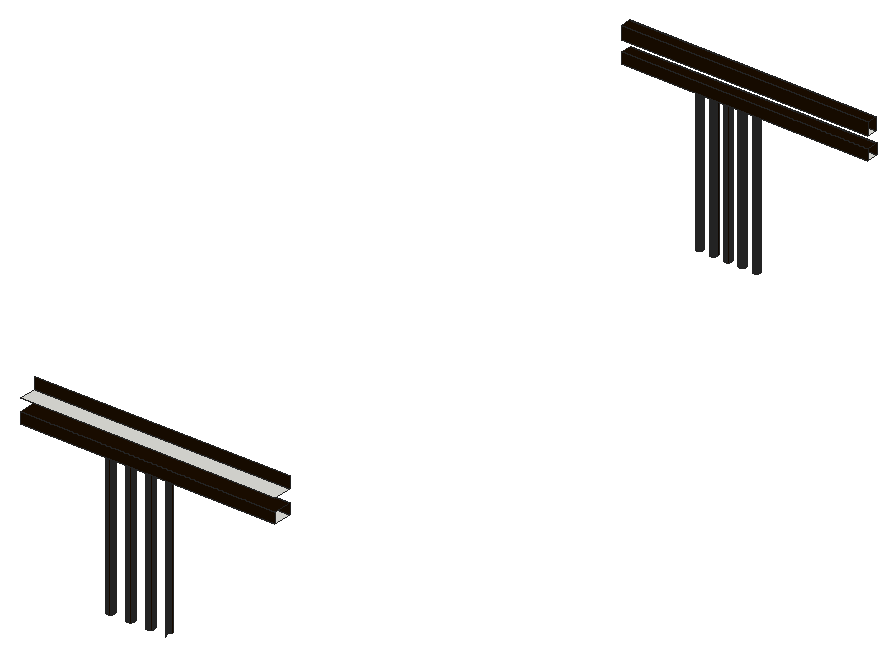
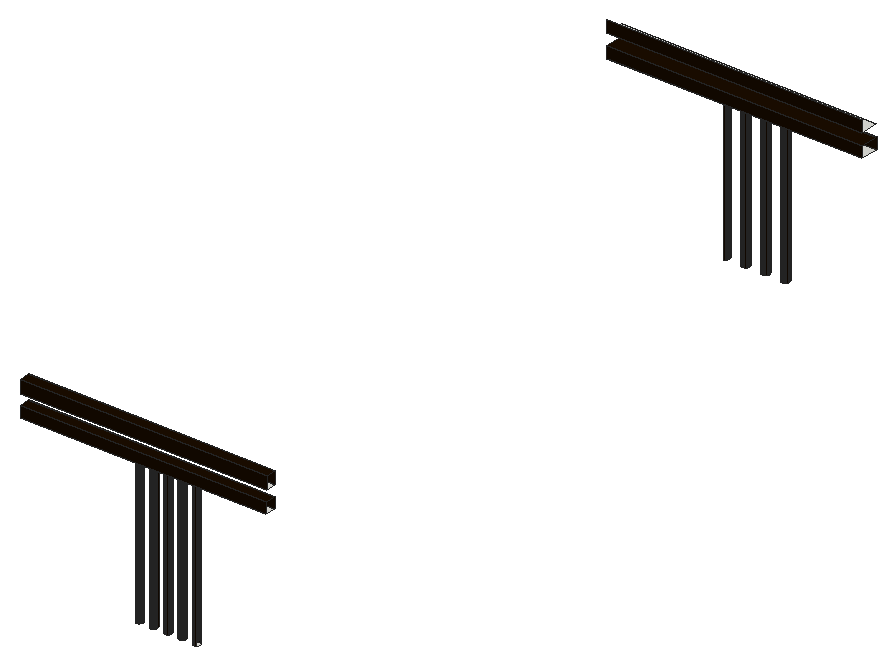
# SketchUp Ruby script. Lengths in inches.
U = 1.inch
M = Sketchup.active_model
def pt(a) = Geom::Point3d.new(a.map { |v| v * U })
def face(e, loops, mat)
  f = e.add_face(loops[0].map { |a| pt(a) })
  loops[1..].each { |l| e.add_face(l.map { |a| pt(a) }).erase! }
  f.material = f.back_material = mat if mat
  f
end
# faces: each face lists its corners as indices into pts; further lists are holes
def faces(e, pts, list, mat = nil) = list.each { |f| face(e, (f[0].is_a?(Array) ? f : [f]).map { |l| l.map { |i| pts[i] } }, mat) }
# xy, xz, yz: faces in a plane at the given z, y or x. An outline is a flat list of corners, or four numbers for a rectangle; further outlines are holes
def ring(l) = l.size == 4 ? [[l[0], l[1]], [l[2], l[1]], [l[2], l[3]], [l[0], l[3]]] : l.each_slice(2).to_a
def flat(e, list, mat, &to3) = list.each { |f| face(e, (f[0].is_a?(Array) ? f : [f]).map { |l| ring(l).map { |u, v| to3.(u, v) } }, mat) }
def xy(e, z, list, mat = nil) = flat(e, list, mat) { |x, y| [x, y, z] }
def xz(e, y, list, mat = nil) = flat(e, list, mat) { |x, z| [x, y, z] }
def yz(e, x, list, mat = nil) = flat(e, list, mat) { |y, z| [x, y, z] }
def lines(e, pts, list) = list.each { |a, b| e.add_line(pt(pts[a]), pt(pts[b])) }
# prism: a flat outline (further loops are holes) pulled along v
def prism(e, loops, v, mat = nil)
  f = face(e, loops, mat); d = Geom::Vector3d.new(v.map { |x| x * U })
  f.pushpull(f.normal.samedirection?(d) ? d.length : -d.length)
end
def box(e, o, s, mat = nil) = prism(e, [[o, [o[0] + s[0], o[1], o[2]], [o[0] + s[0], o[1] + s[1], o[2]], [o[0], o[1] + s[1], o[2]]]], [0, 0, s[2]], mat)
def at(x, y, z, deg = 0) = Geom::Transformation.translation(pt([x, y, z])) * Geom::Transformation.rotation(ORIGIN, Z_AXIS, deg.degrees)
def axes(o, x, y, z) = Geom::Transformation.new([*x, 0, *y, 0, *z, 0, *pt(o).to_a, 1])
def part(name) = M.definitions.add(name)
# library, detail: a bought-in or finely detailed component or shape, given as its bounding box
def library(name, o, s) = part(name).tap { |d| box(d.entities, o, s) }
def detail(e, o, s) = box(e.add_group.entities, o, s)
def put(e, d, t, mat = nil) = e.add_instance(d, t).tap { |i| i.material = mat if mat }
def group(e, t, mat = nil) = e.add_group.tap { |g| g.transformation = t; g.material = mat if mat }.entities
root = M.entities
M.materials.add("[Metal Seamed]1").color = [28, 14, 0]
xy(root,618.25,[[304.26,68.79,303.92,68.83,303.61,68.97,303.33,69.17,303.125,69.45,302.99,69.76,302.95,70.1,302.99,70.44,303.125,70.76,303.33,71.03,303.61,71.24,303.92,71.37,304.26,71.41,304.6,71.37,304.92,71.24,305.19,71.03,305.4,70.76,305.53,70.44,305.57,70.1,305.53,69.76,305.4,69.45,305.19,69.17,304.92,68.97,304.6,68.83],[310.95,68.79,310.61,68.83,310.29,68.97,310.02,69.17,309.8125,69.45,309.68,69.76,309.64,70.1,309.68,70.44,309.8125,70.76,310.02,71.03,310.29,71.24,310.61,71.37,310.95,71.41,311.29,71.37,311.61,71.24,311.88,71.03,312.09,70.76,312.22,70.44,312.26,70.1,312.22,69.76,312.09,69.45,311.88,69.17,311.61,68.97,311.29,68.83],[303.33,318.74,303.05,318.8125,302.79,318.95,302.57,319.15,302.42,319.4,302.34,319.6875,302.33,319.98,302.4,320.27,302.54,320.52,302.74,320.74,302.99,320.89,303.27,320.97,303.57,320.98,303.85,320.91,304.11,320.77,304.32,320.57,304.48,320.32,304.56,320.04,304.57,319.74,304.5,319.46,304.36,319.2,304.16,318.99,303.91,318.83,303.625,318.75],[308.14,318.74,307.86,318.8125,307.6,318.95,307.39,319.15,307.23,319.4,307.15,319.6875,307.14,319.98,307.21,320.27,307.35,320.52,307.55,320.74,307.8,320.89,308.09,320.97,308.38,320.98,308.66,320.91,308.92,320.77,309.14,320.57,309.29,320.32,309.37,320.04,309.38,319.74,309.3125,319.46,309.17,319.2,308.97,318.99,308.72,318.83,308.4375,318.75],[312.96,318.74,312.67,318.8125,312.41,318.95,312.2,319.15,312.05,319.4,311.96,319.6875,311.96,319.98,312.02,320.27,312.16,320.52,312.37,320.74,312.62,320.89,312.9,320.97,313.19,320.98,313.48,320.91,313.74,320.77,313.95,320.57,314.1,320.32,314.19,320.04,314.19,319.74,314.125,319.46,313.98,319.2,313.78,318.99,313.53,318.83,313.25,318.75],
  [317.77,318.74,317.48,318.8125,317.23,318.95,317.01,319.15,316.86,319.4,316.78,319.6875,316.77,319.98,316.84,320.27,316.98,320.52,317.18,320.74,317.43,320.89,317.71,320.97,318,320.98,318.29,320.91,318.55,320.77,318.76,320.57,318.91,320.32,319,320.04,319.01,319.74,318.9375,319.46,318.8,319.2,318.59,318.99,318.34,318.83,318.0625,318.75],[322.58,318.74,322.3,318.8125,322.04,318.95,321.82,319.15,321.67,319.4,321.59,319.6875,321.58,319.98,321.65,320.27,321.79,320.52,321.99,320.74,322.24,320.89,322.52,320.97,322.82,320.98,323.1,320.91,323.36,320.77,323.57,320.57,323.73,320.32,323.81,320.04,323.82,319.74,323.75,319.46,323.61,319.2,323.41,318.99,323.16,318.83,322.875,318.75]])
xy(root,666.66,[[[275.92,67.16,361.98,73.28],[284.2,68.79,284.54,68.83,284.86,68.97,285.13,69.17,285.34,69.45,285.47,69.76,285.51,70.1,285.47,70.44,285.34,70.76,285.13,71.03,284.86,71.24,284.54,71.37,284.2,71.41,283.86,71.37,283.54,71.24,283.27,71.03,283.0625,70.76,282.93,70.44,282.89,70.1,282.93,69.76,283.0625,69.45,283.27,69.17,283.54,68.97,283.86,68.83],[290.89,68.79,291.23,68.83,291.54,68.97,291.81,69.17,292.02,69.45,292.15,69.76,292.2,70.1,292.15,70.44,292.02,70.76,291.81,71.03,291.54,71.24,291.23,71.37,290.89,71.41,290.55,71.37,290.23,71.24,289.96,71.03,289.75,70.76,289.62,70.44,289.57,70.1,289.62,69.76,289.75,69.45,289.96,69.17,290.23,68.97,290.55,68.83],[297.57,68.79,297.91,68.83,298.23,68.97,298.5,69.17,298.71,69.45,298.84,69.76,298.89,70.1,298.84,70.44,298.71,70.76,298.5,71.03,298.23,71.24,297.91,71.37,297.57,71.41,297.23,71.37,296.92,71.24,296.65,71.03,296.4375,70.76,296.31,70.44,296.26,70.1,296.31,69.76,296.4375,69.45,296.65,69.17,296.92,68.97,297.23,68.83],[304.26,68.79,304.6,68.83,304.92,68.97,305.19,69.17,305.4,69.45,305.53,69.76,305.57,70.1,305.53,70.44,305.4,70.76,305.19,71.03,304.92,71.24,304.6,71.37,304.26,71.41,303.92,71.37,303.61,71.24,303.33,71.03,303.125,70.76,302.99,70.44,302.95,70.1,302.99,69.76,303.125,69.45,303.33,69.17,303.61,68.97,303.92,68.83],[310.95,68.79,311.29,68.83,311.61,68.97,311.88,69.17,312.09,69.45,312.22,69.76,312.26,70.1,312.22,70.44,312.09,70.76,311.88,71.03,311.61,71.24,311.29,71.37,310.95,71.41,310.61,71.37,310.29,71.24,310.02,71.03,309.8125,70.76,309.68,70.44,309.64,70.1,309.68,69.76,309.8125,69.45,310.02,69.17,310.29,68.97,310.61,68.83],[324.32,68.79,324.66,68.83,324.98,68.97,325.25,69.17,325.46,69.45,325.59,69.76,325.64,70.1,325.59,70.44,325.46,70.76,325.25,71.03,324.98,71.24,324.66,71.37,324.32,71.41,323.98,71.37,323.67,71.24,323.4,71.03,323.1875,70.76,323.06,70.44,323.01,70.1,323.06,69.76,323.1875,69.45,323.4,69.17,323.67,68.97,323.98,68.83],[331.01,68.79,331.35,68.83,331.67,68.97,331.94,69.17,332.15,69.45,332.28,69.76,332.32,70.1,332.28,70.44,332.15,70.76,331.94,71.03,331.67,71.24,331.35,71.37,331.01,71.41,330.67,71.37,330.36,71.24,330.08,71.03,329.875,70.76,329.74,70.44,329.7,70.1,329.74,69.76,329.875,69.45,330.08,69.17,330.36,68.97,330.67,68.83],[351.89,68.79,352.23,68.83,352.55,68.97,352.82,69.17,353.03,69.45,353.16,69.76,353.2,70.1,353.16,70.44,353.03,70.76,352.82,71.03,352.55,71.24,352.23,71.37,351.89,71.41,351.55,71.37,351.23,71.24,350.96,71.03,350.75,70.76,350.62,70.44,350.58,70.1,350.62,69.76,350.75,69.45,350.96,69.17,351.23,68.97,351.55,68.83],[317.64,68.79,317.98,68.83,318.29,68.97,318.56,69.17,318.77,69.45,318.9,69.76,318.95,70.1,318.9,70.44,318.77,70.76,318.56,71.03,318.29,71.24,317.98,71.37,317.64,71.41,317.3,71.37,316.98,71.24,316.71,71.03,316.5,70.76,316.37,70.44,316.32,70.1,316.37,69.76,316.5,69.45,316.71,69.17,316.98,68.97,317.3,68.83]],[[278.88,317.52,361.98,321.28],[351.46,318.74,351.75,318.75,352.03,318.83,352.28,318.99,352.48,319.2,352.625,319.46,352.69,319.74,352.69,320.04,352.6,320.32,352.45,320.57,352.24,320.77,351.98,320.91,351.69,320.98,351.4,320.97,351.12,320.89,350.87,320.74,350.66,320.52,350.52,320.27,350.46,319.98,350.46,319.6875,350.55,319.4,350.7,319.15,350.91,318.95,351.17,318.8125],[322.58,318.74,322.875,318.75,323.16,318.83,323.41,318.99,323.61,319.2,323.75,319.46,323.82,319.74,323.81,320.04,323.73,320.32,323.57,320.57,323.36,320.77,323.1,320.91,322.82,320.98,322.52,320.97,322.24,320.89,321.99,320.74,321.79,320.52,321.65,320.27,321.58,319.98,321.59,319.6875,321.67,319.4,321.82,319.15,322.04,318.95,322.3,318.8125],[317.77,318.74,318.0625,318.75,318.34,318.83,318.59,318.99,318.8,319.2,318.9375,319.46,319.01,319.74,319,320.04,318.91,320.32,318.76,320.57,318.55,320.77,318.29,320.91,318,320.98,317.71,320.97,317.43,320.89,317.18,320.74,316.98,320.52,316.84,320.27,316.77,319.98,316.78,319.6875,316.86,319.4,317.01,319.15,317.23,318.95,317.48,318.8125],[312.96,318.74,313.25,318.75,313.53,318.83,313.78,318.99,313.98,319.2,314.125,319.46,314.19,319.74,314.19,320.04,314.1,320.32,313.95,320.57,313.74,320.77,313.48,320.91,313.19,320.98,312.9,320.97,312.62,320.89,312.37,320.74,312.16,320.52,312.02,320.27,311.96,319.98,311.96,319.6875,312.05,319.4,312.2,319.15,312.41,318.95,312.67,318.8125],[308.14,318.74,308.4375,318.75,308.72,318.83,308.97,318.99,309.17,319.2,309.3125,319.46,309.38,319.74,309.37,320.04,309.29,320.32,309.14,320.57,308.92,320.77,308.66,320.91,308.38,320.98,308.09,320.97,307.8,320.89,307.55,320.74,307.35,320.52,307.21,320.27,307.14,319.98,307.15,319.6875,307.23,319.4,307.39,319.15,307.6,318.95,307.86,318.8125],[298.52,318.74,298.8125,318.75,299.09,318.83,299.34,318.99,299.55,319.2,299.6875,319.46,299.76,319.74,299.75,320.04,299.66,320.32,299.51,320.57,299.3,320.77,299.04,320.91,298.75,320.98,298.46,320.97,298.18,320.89,297.93,320.74,297.73,320.52,297.59,320.27,297.52,319.98,297.53,319.6875,297.61,319.4,297.76,319.15,297.98,318.95,298.23,318.8125],[293.71,318.74,294,318.75,294.28,318.83,294.53,318.99,294.73,319.2,294.875,319.46,294.94,319.74,294.94,320.04,294.85,320.32,294.7,320.57,294.49,320.77,294.23,320.91,293.94,320.98,293.65,320.97,293.37,320.89,293.12,320.74,292.91,320.52,292.77,320.27,292.71,319.98,292.71,319.6875,292.8,319.4,292.95,319.15,293.16,318.95,293.42,318.8125],[284.08,318.74,284.375,318.75,284.66,318.83,284.91,318.99,285.11,319.2,285.25,319.46,285.32,319.74,285.31,320.04,285.23,320.32,285.07,320.57,284.86,320.77,284.6,320.91,284.32,320.98,284.02,320.97,283.74,320.89,283.49,320.74,283.29,320.52,283.15,320.27,283.08,319.98,283.09,319.6875,283.17,319.4,283.32,319.15,283.54,318.95,283.8,318.8125]]])
xy(root,666.9375,[[303.33,318.74,303.625,318.75,303.91,318.83,304.16,318.99,304.36,319.2,304.5,319.46,304.57,319.74,304.56,320.04,304.48,320.32,304.32,320.57,304.11,320.77,303.85,320.91,303.57,320.98,303.27,320.97,302.99,320.89,302.74,320.74,302.54,320.52,302.4,320.27,302.33,319.98,302.34,319.6875,302.42,319.4,302.57,319.15,302.79,318.95,303.05,318.8125]])
xy(root,670.37,[[275.92,67.16,361.98,73.28],[278.88,317.52,361.98,321.28]],"[Metal Seamed]1")
xy(root,674.05,[[278.82,317.52,361.97,321.28]])
xy(root,674.375,[[275.92,67.28,361.97,73.28]])
xy(root,678.3125,[[278.82,317.52,361.97,321.28]],"[Metal Seamed]1")
xz(root,67.16,[[275.92,666.66,361.98,670.37]],"[Metal Seamed]1")
xz(root,73.28,[[275.92,666.66,361.97,670.37],[275.92,674.375,361.97,678.3125]],"[Metal Seamed]1")
xz(root,317.52,[[278.88,666.66,361.98,670.37],[278.82,674.05,361.97,678.3125]],"[Metal Seamed]1")
xz(root,321.28,[[278.88,666.66,361.98,670.37],[278.82,674.05,361.97,678.3125]],"[Metal Seamed]1")
yz(root,311.96,[[319.6875,618.25,319.98,666.66]],"[Metal Seamed]1")
yz(root,314.19,[[319.74,618.25,320.04,666.66]],"[Metal Seamed]1")
p = [[303.61,68.97,618.25],[303.92,68.83,618.25],[303.92,68.83,666.66],[303.61,68.97,666.66],[304.26,68.79,618.25],[304.26,68.79,666.66],
  [304.6,68.83,618.25],[304.6,68.83,666.66],[304.92,68.97,618.25],[304.92,68.97,666.66],[310.29,68.97,618.25],[310.61,68.83,618.25],
  [310.61,68.83,666.66],[310.29,68.97,666.66],[310.95,68.79,618.25],[310.95,68.79,666.66],[311.29,68.83,618.25],[311.29,68.83,666.66],
  [311.61,68.97,618.25],[311.61,68.97,666.66],[316.98,68.97,618.25],[317.3,68.83,618.25],[317.3,68.83,666.66],[316.98,68.97,666.66],
  [317.64,68.79,618.25],[317.64,68.79,666.66],[317.98,68.83,618.25],[317.98,68.83,666.66],[318.29,68.97,618.25],[318.29,68.97,666.66],
  [303.33,69.17,618.25],[303.33,69.17,666.66],[305.19,69.17,618.25],[305.19,69.17,666.66],[310.02,69.17,618.25],[310.02,69.17,666.66],
  [311.88,69.17,618.25],[311.88,69.17,666.66],[316.71,69.17,618.25],[316.71,69.17,666.66],[318.56,69.17,618.25],[318.56,69.17,666.66],
  [323.4,69.17,618.25],[323.67,68.97,618.25],[323.67,68.97,666.66],[323.4,69.17,666.66],[303.125,69.45,618.25],[303.125,69.45,666.66],
  [305.4,69.45,618.25],[305.4,69.45,666.66],[309.8125,69.45,618.25],[309.8125,69.45,666.66],[312.09,69.45,618.25],[312.09,69.45,666.66],
  [316.5,69.45,618.25],[316.5,69.45,666.66],[318.77,69.45,618.25],[318.77,69.45,666.66],[323.1875,69.45,618.25],[323.1875,69.45,666.66],
  [302.99,69.76,618.25],[302.99,69.76,666.66],[305.53,69.76,618.25],[305.53,69.76,666.66],[309.68,69.76,618.25],[309.68,69.76,666.66],
  [312.22,69.76,618.25],[312.22,69.76,666.66],[316.37,69.76,618.25],[316.37,69.76,666.66],[318.9,69.76,618.25],[318.9,69.76,666.66],
  [323.06,69.76,618.25],[323.06,69.76,666.66],[302.95,70.1,618.25],[302.95,70.1,666.66],[305.57,70.1,618.25],[305.57,70.1,666.66],
  [309.64,70.1,618.25],[309.64,70.1,666.66],[312.26,70.1,618.25],[312.26,70.1,666.66],[316.32,70.1,618.25],[316.32,70.1,666.66],
  [318.95,70.1,618.25],[318.95,70.1,666.66],[323.01,70.1,618.25],[323.01,70.1,666.66],[302.99,70.44,618.25],[302.99,70.44,666.66],
  [305.53,70.44,618.25],[305.53,70.44,666.66],[309.68,70.44,618.25],[309.68,70.44,666.66],[312.22,70.44,618.25],[312.22,70.44,666.66],
  [316.37,70.44,618.25],[316.37,70.44,666.66],[318.9,70.44,618.25],[318.9,70.44,666.66],[323.06,70.44,618.25],[323.06,70.44,666.66],
  [303.125,70.76,618.25],[303.125,70.76,666.66],[305.4,70.76,618.25],[305.4,70.76,666.66],[309.8125,70.76,618.25],[309.8125,70.76,666.66],
  [312.09,70.76,618.25],[312.09,70.76,666.66],[316.5,70.76,618.25],[316.5,70.76,666.66],[318.77,70.76,618.25],[318.77,70.76,666.66],
  [323.1875,70.76,618.25],[323.1875,70.76,666.66],[303.33,71.03,618.25],[303.33,71.03,666.66],[305.19,71.03,618.25],[305.19,71.03,666.66],
  [310.02,71.03,618.25],[310.02,71.03,666.66],[311.88,71.03,618.25],[311.88,71.03,666.66],[316.71,71.03,618.25],[316.71,71.03,666.66],
  [318.56,71.03,618.25],[318.56,71.03,666.66],[323.4,71.03,618.25],[323.4,71.03,666.66],[303.61,71.24,618.25],[303.61,71.24,666.66],
  [304.92,71.24,618.25],[304.92,71.24,666.66],[310.29,71.24,618.25],[310.29,71.24,666.66],[311.61,71.24,618.25],[311.61,71.24,666.66],
  [316.98,71.24,618.25],[316.98,71.24,666.66],[318.29,71.24,618.25],[318.29,71.24,666.66],[323.67,71.24,618.25],[323.67,71.24,666.66],
  [303.92,71.37,618.25],[303.92,71.37,666.66],[304.6,71.37,618.25],[304.6,71.37,666.66],[310.61,71.37,618.25],[310.61,71.37,666.66],
  [311.29,71.37,618.25],[311.29,71.37,666.66],[317.3,71.37,618.25],[317.3,71.37,666.66],[317.98,71.37,618.25],[317.98,71.37,666.66],
  [323.98,71.37,618.25],[323.98,71.37,666.66],[304.26,71.41,618.25],[304.26,71.41,666.66],[310.95,71.41,618.25],[310.95,71.41,666.66],
  [317.64,71.41,618.25],[317.64,71.41,666.66],[303.05,318.8125,618.25],[303.33,318.74,618.25],[303.33,318.74,666.9375],[303.05,318.8125,666.9375],
  [303.625,318.75,618.25],[303.625,318.75,666.9375],[307.86,318.8125,618.25],[308.14,318.74,618.25],[308.14,318.74,666.66],[307.86,318.8125,666.66],
  [308.4375,318.75,618.25],[308.4375,318.75,666.66],[312.67,318.8125,618.25],[312.96,318.74,618.25],[312.96,318.74,666.66],[312.67,318.8125,666.66],
  [313.25,318.75,618.25],[313.25,318.75,666.66],[317.48,318.8125,618.25],[317.77,318.74,618.25],[317.77,318.74,666.66],[317.48,318.8125,666.66],
  [318.0625,318.75,618.25],[318.0625,318.75,666.66],[322.3,318.8125,618.25],[322.58,318.74,618.25],[322.58,318.74,666.66],[322.3,318.8125,666.66],
  [322.875,318.75,618.25],[322.875,318.75,666.66],[303.91,318.83,618.25],[303.91,318.83,666.9375],[304.16,318.99,618.25],[304.16,318.99,666.9375],
  [307.6,318.95,618.25],[307.6,318.95,666.66],[308.72,318.83,618.25],[308.72,318.83,666.66],[308.97,318.99,618.25],[308.97,318.99,666.66],
  [312.41,318.95,618.25],[312.41,318.95,666.66],[313.53,318.83,618.25],[313.53,318.83,666.66],[313.78,318.99,618.25],[313.78,318.99,666.66],
  [317.23,318.95,618.25],[317.23,318.95,666.66],[318.34,318.83,618.25],[318.34,318.83,666.66],[318.59,318.99,618.25],[318.59,318.99,666.66],
  [322.04,318.95,618.25],[322.04,318.95,666.66],[323.16,318.83,618.25],[323.16,318.83,666.66],[323.41,318.99,618.25],[323.41,318.99,666.66],
  [304.36,319.2,618.25],[304.36,319.2,666.9375],[307.39,319.15,618.25],[307.39,319.15,666.66],[309.17,319.2,618.25],[309.17,319.2,666.66],
  [312.2,319.15,618.25],[312.2,319.15,666.66],[313.98,319.2,618.25],[313.98,319.2,666.66],[317.01,319.15,618.25],[317.01,319.15,666.66],
  [318.8,319.2,618.25],[318.8,319.2,666.66],[321.82,319.15,618.25],[321.82,319.15,666.66],[323.61,319.2,618.25],[323.61,319.2,666.66],
  [304.5,319.46,618.25],[304.5,319.46,666.9375],[307.23,319.4,618.25],[307.23,319.4,666.66],[309.3125,319.46,618.25],[309.3125,319.46,666.66],
  [312.05,319.4,618.25],[312.05,319.4,666.66],[314.125,319.46,618.25],[314.125,319.46,666.66],[316.86,319.4,618.25],[316.86,319.4,666.66],
  [318.9375,319.46,618.25],[318.9375,319.46,666.66],[321.67,319.4,618.25],[321.67,319.4,666.66],[323.75,319.46,618.25],[323.75,319.46,666.66],
  [307.15,319.6875,618.25],[307.15,319.6875,666.66],[311.96,319.6875,618.25],[311.96,319.6875,666.66],[316.78,319.6875,618.25],[316.78,319.6875,666.66],
  [321.59,319.6875,618.25],[321.59,319.6875,666.66],[304.57,319.74,618.25],[304.57,319.74,666.9375],[309.38,319.74,618.25],[309.38,319.74,666.66],
  [314.19,319.74,618.25],[314.19,319.74,666.66],[319.01,319.74,618.25],[319.01,319.74,666.66],[323.82,319.74,618.25],[323.82,319.74,666.66],
  [304.56,320.04,618.25],[304.56,320.04,666.9375],[307.14,319.98,618.25],[307.14,319.98,666.66],[309.37,320.04,618.25],[309.37,320.04,666.66],
  [316.77,319.98,618.25],[316.77,319.98,666.66],[319,320.04,618.25],[319,320.04,666.66],[321.58,319.98,618.25],[321.58,319.98,666.66],
  [323.81,320.04,618.25],[323.81,320.04,666.66],[304.48,320.32,618.25],[304.48,320.32,666.9375],[307.21,320.27,618.25],[307.21,320.27,666.66],
  [309.29,320.32,618.25],[309.29,320.32,666.66],[312.02,320.27,618.25],[311.96,319.98,618.25],[311.96,319.98,666.66],[312.02,320.27,666.66],
  [314.19,320.04,618.25],[314.1,320.32,618.25],[314.1,320.32,666.66],[314.19,320.04,666.66],[316.84,320.27,618.25],[316.84,320.27,666.66],
  [318.91,320.32,618.25],[318.91,320.32,666.66],[321.65,320.27,618.25],[321.65,320.27,666.66],[323.73,320.32,618.25],[323.73,320.32,666.66],
  [304.32,320.57,618.25],[304.32,320.57,666.9375],[307.35,320.52,618.25],[307.35,320.52,666.66],[309.14,320.57,618.25],[309.14,320.57,666.66],
  [312.16,320.52,618.25],[312.16,320.52,666.66],[313.95,320.57,618.25],[313.95,320.57,666.66],[316.98,320.52,618.25],[316.98,320.52,666.66],
  [318.76,320.57,618.25],[318.76,320.57,666.66],[321.79,320.52,618.25],[321.79,320.52,666.66],[323.57,320.57,618.25],[323.57,320.57,666.66],
  [307.55,320.74,618.25],[307.55,320.74,666.66],[312.37,320.74,618.25],[312.37,320.74,666.66],[317.18,320.74,618.25],[317.18,320.74,666.66],
  [321.99,320.74,618.25],[321.99,320.74,666.66],[304.11,320.77,618.25],[304.11,320.77,666.9375],[308.92,320.77,618.25],[308.92,320.77,666.66],
  [313.74,320.77,618.25],[313.74,320.77,666.66],[318.55,320.77,618.25],[318.55,320.77,666.66],[323.36,320.77,618.25],[323.36,320.77,666.66],
  [307.8,320.89,618.25],[307.8,320.89,666.66],[312.62,320.89,618.25],[312.62,320.89,666.66],[317.43,320.89,618.25],[317.43,320.89,666.66],
  [322.24,320.89,618.25],[322.24,320.89,666.66],[303.85,320.91,618.25],[303.85,320.91,666.9375],[308.66,320.91,618.25],[308.66,320.91,666.66],
  [313.48,320.91,618.25],[313.48,320.91,666.66],[318.29,320.91,618.25],[318.29,320.91,666.66],[323.1,320.91,618.25],[323.1,320.91,666.66],
  [303.27,320.97,618.25],[302.99,320.89,618.25],[302.99,320.89,666.9375],[303.27,320.97,666.9375],[303.57,320.98,618.25],[303.57,320.98,666.9375],
  [308.09,320.97,618.25],[308.09,320.97,666.66],[308.38,320.98,618.25],[308.38,320.98,666.66],[312.9,320.97,618.25],[312.9,320.97,666.66],
  [313.19,320.98,618.25],[313.19,320.98,666.66],[317.71,320.97,618.25],[317.71,320.97,666.66],[318,320.98,618.25],[318,320.98,666.66],
  [322.52,320.97,618.25],[322.52,320.97,666.66],[322.82,320.98,618.25],[322.82,320.98,666.66]]
faces(root,p,[[0,1,2,3],[1,4,5,2],[4,6,7,5],[6,8,9,7],[10,11,12,13],[11,14,15,12],[14,16,17,15],[16,18,19,17],
  [20,21,22,23],[21,24,25,22],[24,26,27,25],[26,28,29,27],[30,0,3,31],[8,32,33,9],[34,10,13,35],[18,36,37,19],
  [38,20,23,39],[28,40,41,29],[42,43,44,45],[46,30,31,47],[32,48,49,33],[50,34,35,51],[36,52,53,37],[54,38,39,55],
  [40,56,57,41],[58,42,45,59],[60,46,47,61],[48,62,63,49],[64,50,51,65],[52,66,67,53],[68,54,55,69],[56,70,71,57],
  [72,58,59,73],[74,60,61,75],[62,76,77,63],[78,64,65,79],[66,80,81,67],[82,68,69,83],[70,84,85,71],[86,72,73,87],
  [88,74,75,89],[76,90,91,77],[92,78,79,93],[80,94,95,81],[96,82,83,97],[84,98,99,85],[100,86,87,101],[102,88,89,103],
  [90,104,105,91],[106,92,93,107],[94,108,109,95],[110,96,97,111],[98,112,113,99],[114,100,101,115],[116,102,103,117],[104,118,119,105],
  [120,106,107,121],[108,122,123,109],[124,110,111,125],[112,126,127,113],[128,114,115,129],[130,116,117,131],[118,132,133,119],[134,120,121,135],
  [122,136,137,123],[138,124,125,139],[126,140,141,127],[142,128,129,143],[144,130,131,145],[132,146,147,133],[148,134,135,149],[136,150,151,137],
  [152,138,139,153],[140,154,155,141],[156,142,143,157],[158,144,145,159],[146,158,159,147],[160,148,149,161],[150,160,161,151],[162,152,153,163],
  [154,162,163,155],[164,165,166,167],[165,168,169,166],[170,171,172,173],[171,174,175,172],[176,177,178,179],[177,180,181,178],[182,183,184,185],
  [183,186,187,184],[188,189,190,191],[189,192,193,190],[168,194,195,169],[194,196,197,195],[198,170,173,199],[174,200,201,175],[200,202,203,201],
  [204,176,179,205],[180,206,207,181],[206,208,209,207],[210,182,185,211],[186,212,213,187],[212,214,215,213],[216,188,191,217],[192,218,219,193],
  [218,220,221,219],[196,222,223,197],[224,198,199,225],[202,226,227,203],[228,204,205,229],[208,230,231,209],[232,210,211,233],[214,234,235,215],
  [236,216,217,237],[220,238,239,221],[222,240,241,223],[242,224,225,243],[226,244,245,227],[246,228,229,247],[230,248,249,231],[250,232,233,251],
  [234,252,253,235],[254,236,237,255],[238,256,257,239],[258,242,243,259],[260,246,247,261],[262,250,251,263],[264,254,255,265],[240,266,267,241],
  [244,268,269,245],[248,270,271,249],[252,272,273,253],[256,274,275,257],[266,276,277,267],[278,258,259,279],[268,280,281,269],[282,262,263,283],
  [272,284,285,273],[286,264,265,287],[274,288,289,275],[276,290,291,277],[292,278,279,293],[280,294,295,281],[296,297,298,299],[300,301,302,303],
  [304,282,283,305],[284,306,307,285],[308,286,287,309],[288,310,311,289],[290,312,313,291],[314,292,293,315],[294,316,317,295],[318,296,299,319],
  [301,320,321,302],[322,304,305,323],[306,324,325,307],[326,308,309,327],[310,328,329,311],[330,314,315,331],[332,318,319,333],[334,322,323,335],
  [336,326,327,337],[312,338,339,313],[316,340,341,317],[320,342,343,321],[324,344,345,325],[328,346,347,329],[348,330,331,349],[350,332,333,351],
  [352,334,335,353],[354,336,337,355],[338,356,357,339],[340,358,359,341],[342,360,361,343],[344,362,363,345],[346,364,365,347],[366,367,368,369],
  [356,370,371,357],[372,348,349,373],[358,374,375,359],[376,350,351,377],[360,378,379,361],[380,352,353,381],[362,382,383,363],[384,354,355,385],
  [364,386,387,365],[370,366,369,371],[374,372,373,375],[378,376,377,379],[382,380,381,383],[386,384,385,387]],"[Metal Seamed]1")
